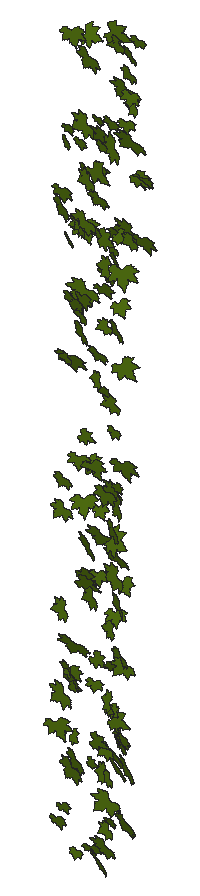
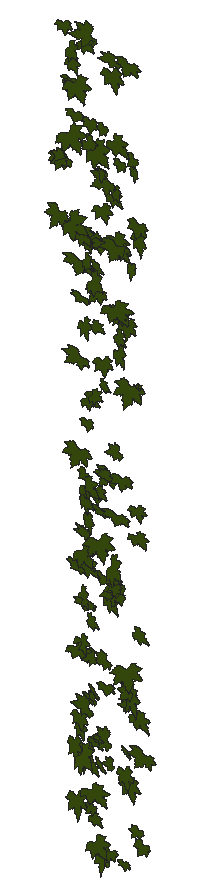
# SketchUp Ruby script. Lengths in inches.
U = 1.inch
M = Sketchup.active_model
def pt(a) = Geom::Point3d.new(a.map { |v| v * U })
def face(e, loops, mat)
  f = e.add_face(loops[0].map { |a| pt(a) })
  loops[1..].each { |l| e.add_face(l.map { |a| pt(a) }).erase! }
  f.material = f.back_material = mat if mat
  f
end
# faces: each face lists its corners as indices into pts; further lists are holes
def faces(e, pts, list, mat = nil) = list.each { |f| face(e, (f[0].is_a?(Array) ? f : [f]).map { |l| l.map { |i| pts[i] } }, mat) }
# xy, xz, yz: faces in a plane at the given z, y or x. An outline is a flat list of corners, or four numbers for a rectangle; further outlines are holes
def ring(l) = l.size == 4 ? [[l[0], l[1]], [l[2], l[1]], [l[2], l[3]], [l[0], l[3]]] : l.each_slice(2).to_a
def flat(e, list, mat, &to3) = list.each { |f| face(e, (f[0].is_a?(Array) ? f : [f]).map { |l| ring(l).map { |u, v| to3.(u, v) } }, mat) }
def xy(e, z, list, mat = nil) = flat(e, list, mat) { |x, y| [x, y, z] }
def xz(e, y, list, mat = nil) = flat(e, list, mat) { |x, z| [x, y, z] }
def yz(e, x, list, mat = nil) = flat(e, list, mat) { |y, z| [x, y, z] }
def lines(e, pts, list) = list.each { |a, b| e.add_line(pt(pts[a]), pt(pts[b])) }
# prism: a flat outline (further loops are holes) pulled along v
def prism(e, loops, v, mat = nil)
  f = face(e, loops, mat); d = Geom::Vector3d.new(v.map { |x| x * U })
  f.pushpull(f.normal.samedirection?(d) ? d.length : -d.length)
end
def box(e, o, s, mat = nil) = prism(e, [[o, [o[0] + s[0], o[1], o[2]], [o[0] + s[0], o[1] + s[1], o[2]], [o[0], o[1] + s[1], o[2]]]], [0, 0, s[2]], mat)
def at(x, y, z, deg = 0) = Geom::Transformation.translation(pt([x, y, z])) * Geom::Transformation.rotation(ORIGIN, Z_AXIS, deg.degrees)
def axes(o, x, y, z) = Geom::Transformation.new([*x, 0, *y, 0, *z, 0, *pt(o).to_a, 1])
def part(name) = M.definitions.add(name)
# library, detail: a bought-in or finely detailed component or shape, given as its bounding box
def library(name, o, s) = part(name).tap { |d| box(d.entities, o, s) }
def detail(e, o, s) = box(e.add_group.entities, o, s)
def put(e, d, t, mat = nil) = e.add_instance(d, t).tap { |i| i.material = mat if mat }
def group(e, t, mat = nil) = e.add_group.tap { |g| g.transformation = t; g.material = mat if mat }.entities
root = M.entities
M.materials.add("[Vegetation Blur 03]").color = [83, 114, 18]
c1 = part("ivy")
xy(c1.entities,0,[[0.782,0,0.786,0,0.787,0.005,0.789,0.009,0.821,0.072,0.875,0.147,1.001,0.272,1.073,0.331,1.137,0.363,1.178,0.379,1.223,0.384,1.272,0.383,1.311,0.374,1.36,0.355,1.399,0.334,1.491,0.285,1.541,0.244,1.583,0.199,1.617,0.15,1.64,0.128,1.662,0.115,1.717,0.105,1.745,0.093,1.784,0.054,1.819,0.057,1.854,0.064,1.882,0.075,1.896,0.074,1.91,0.071,1.937,0.063,1.964,0.053,1.99,0.038,2.016,0.015,2.034,0.002,2.04,0,2.038,0.003,2.036,0.007,2.033,0.038,2.036,0.068,2.045,0.1,2.055,0.116,2.064,0.123,2.077,0.129,2.088,0.129,2.106,0.132,2.118,0.13,2.179,0.132,2.207,0.133,2.225,0.133,2.242,0.138,2.22,0.162,2.207,0.186,2.206,0.213,2.212,0.236,2.228,0.262,2.247,0.274,2.298,0.283,2.355,0.294,2.37,0.296,2.376,0.295,2.377,0.3,2.377,0.303,2.385,0.329,2.411,0.37,2.426,0.392,2.449,0.407,2.511,0.426,2.561,0.444,2.619,0.466,2.589,0.469,2.561,0.476,2.501,0.5,2.449,0.516,2.424,0.523,2.401,0.535,2.377,0.556,2.372,0.568,2.36,0.575,2.268,0.586,2.225,0.592,2.207,0.599,2.194,0.61,2.143,0.65,2.13,0.664,2.122,0.682,2.123,0.7,2.13,0.719,2.148,0.75,2.17,0.781,2.195,0.807,2.221,0.828,2.284,0.874,2.291,0.88,2.288,0.887,2.276,0.9,2.267,0.916,2.265,0.933,2.273,0.967,2.292,1.002,2.313,1.03,2.334,1.054,2.348,1.067,2.358,1.074,2.363,1.076,2.362,1.081,2.35,1.094,2.347,1.11,2.35,1.143,2.359,1.18,2.385,1.254,2.415,1.324,2.448,1.393,2.45,1.4,2.446,1.398,2.44,1.394,2.427,1.383,2.402,1.36,2.376,1.339,2.345,1.324,2.305,1.309,2.282,1.303,2.273,1.306,2.245,1.294,2.212,1.287,2.187,1.291,2.163,1.301,2.142,1.316,2.134,1.327,2.124,1.325,2.09,1.292,2.053,1.259,2.014,1.234,1.973,1.215,1.954,1.21,1.931,1.208,1.909,1.212,1.893,1.22,1.879,1.233,1.872,1.248,1.867,1.281,1.864,1.319,1.821,1.258,1.773,1.197,1.726,1.141,1.698,1.121,1.679,1.116,1.666,1.117,1.647,1.122,1.632,1.129,1.62,1.141,1.617,1.154,1.617,1.219,1.621,1.254,1.623,1.268,1.623,1.281,1.618,1.314,1.606,1.346,1.603,1.375,1.607,1.403,1.603,1.467,1.599,1.499,1.605,1.525,1.614,1.552,1.629,1.577,1.635,1.589,1.629,1.587,1.618,1.582,1.596,1.566,1.581,1.556,1.568,1.552,1.557,1.55,1.545,1.553,1.531,1.562,1.522,1.572,1.504,1.591,1.486,1.611,1.474,1.631,1.457,1.666,1.455,1.684,1.457,1.698,1.452,1.715,1.444,1.728,1.424,1.754,1.419,1.772,1.423,1.786,1.434,1.819,1.444,1.848,1.446,1.855,1.44,1.861,1.43,1.867,1.386,1.904,1.349,1.948,1.326,1.973,1.31,1.995,1.288,2.048,1.284,2.153,1.287,2.254,1.284,2.255,1.282,2.253,1.278,2.247,1.274,2.237,1.266,2.216,1.226,2.125,1.208,2.076,1.184,2.033,1.155,1.984,1.135,1.942,1.111,1.899,1.083,1.861,1.053,1.85,1.059,1.83,1.061,1.809,1.056,1.79,1.049,1.767,1.04,1.749,1.018,1.733,0.994,1.726,0.942,1.734,0.95,1.6875,0.944,1.645,0.932,1.608,0.911,1.585,0.881,1.58,0.854,1.582,0.828,1.588,0.785,1.618,0.773,1.625,0.775,1.614,0.779,1.598,0.796,1.502,0.818,1.402,0.861,1.283,0.882,1.224,0.894,1.174,0.892,1.148,0.886,1.123,0.881,1.107,0.872,1.099,0.849,1.094,0.818,1.092,0.789,1.098,0.762,1.107,0.753,1.113,0.721,1.139,0.698,1.163,0.678,1.194,0.665,1.224,0.628,1.28,0.612,1.312,0.606,1.327,0.606,1.314,0.599,1.282,0.594,1.267,0.581,1.256,0.544,1.245,0.512,1.244,0.473,1.249,0.444,1.256,0.382,1.288,0.339,1.306,0.324,1.316,0.317,1.324,0.309,1.326,0.27,1.314,0.227,1.313,0.185,1.3125,0.152,1.317,0.122,1.328,0.092,1.345,0.073,1.353,0.079,1.338,0.092,1.308,0.117,1.249,0.13,1.215,0.139,1.164,0.147,1.148,0.157,1.136,0.163,1.122,0.174,1.086,0.177,1.067,0.182,1.054,0.186,1.043,0.191,1.038,0.211,1.028,0.237,1.005,0.25,0.974,0.253,0.96,0.25,0.944,0.242,0.914,0.243,0.906,0.249,0.902,0.26,0.894,0.289,0.88,0.307,0.873,0.322,0.862,0.364,0.799,0.403,0.738,0.431,0.709,0.439,0.691,0.441,0.678,0.4375,0.66,0.428,0.645,0.394,0.623,0.303,0.594,0.255,0.581,0.214,0.577,0.179,0.573,0.173,0.568,0.175,0.561,0.167,0.55,0.141,0.523,0.113,0.503,0.077,0.49,0.045,0.486,0.026,0.485,0.019,0.486,0.011,0.483,0,0.471,0.014,0.467,0.044,0.455,0.058,0.447,0.07,0.438,0.097,0.411,0.125,0.394,0.158,0.377,0.174,0.366,0.182,0.359,0.185,0.361,0.242,0.331,0.253,0.316,0.258,0.303,0.262,0.283,0.274,0.278,0.308,0.274,0.341,0.252,0.366,0.226,0.366,0.222,0.37,0.22,0.38,0.221,0.395,0.221,0.425,0.216,0.45,0.207,0.465,0.192,0.473,0.178,0.484,0.15,0.489,0.116,0.483,0.089,0.468,0.058,0.45,0.035,0.435,0.018,0.429,0.011,0.434,0.012,0.438,0.014,0.469,0.019,0.542,0.016,0.581,0.015,0.612,0.027,0.68,0.055,0.696,0.057,0.712,0.052,0.73,0.045,0.741,0.036,0.766,0.014]])
p = [[34.46,174.5,46.56],[34.375,174.5,46.56]]
lines(root,p,[[0,1]])
put(root,c1,axes([27.85,173.7,7.37],[0.37849,-0.06704,0.09137],[0.11442,0.06293,-0.30843],[-0.02244,-0.80977,-0.03153]),"[Vegetation Blur 03]")
put(root,c1,axes([27.48,173.7,12.03],[0.53376,0.03726,0.21952],[0.269,0.00727,-0.43585],[0.01776,-1.22992,0.00407]),"[Vegetation Blur 03]")
put(root,c1,axes([28.43,173.7,14.45],[0.42826,-0.11256,-0.35023],[-0.42906,0.04831,-0.35189],[-0.05529,-1.24664,0.01798]),"[Vegetation Blur 03]")
put(root,c1,axes([28.76,173.7,18.72],[0.19822,-0.13225,-0.36337],[-0.44645,0.06503,-0.16594],[-0.0552,-1.0008,0.03723]),"[Vegetation Blur 03]")
put(root,c1,axes([28.37,173.7,23.69],[0.40363,-0.02669,-0.22372],[-0.27442,-0.04788,-0.32887],[0.00236,-1.00289,0.02165]),"[Vegetation Blur 03]")
put(root,c1,axes([28.3,173.7,25.06],[0.38167,-0.01698,-0.15187],[-0.18516,0.0606,-0.31101],[-0.02031,-0.87168,-0.01866]),"[Vegetation Blur 03]")
put(root,c1,axes([28.29,173.7,39.18],[0.47471,-0.2198,-0.23723],[-0.27334,0.21714,-0.39597],[-0.14555,-1.12467,-0.03009]),"[Vegetation Blur 03]")
put(root,c1,axes([28.78,173.7,31.25],[0.13027,0.06294,-0.24641],[-0.30303,0.06322,-0.10416],[-0.01626,-0.67369,-0.0328]),"[Vegetation Blur 03]")
put(root,c1,axes([28.02,173.7,39.6],[0.49002,-0.06773,0.03255],[0.04203,0.06603,-0.39982],[-0.03013,-1.00954,-0.02833]),"[Vegetation Blur 03]")
put(root,c1,axes([28.22,173.7,8.02],[0.2717,-0.01326,0.11926],[0.14597,0.06528,-0.22036],[0.00938,-0.63148,-0.02528]),"[Vegetation Blur 03]")
put(root,c1,axes([28.79,173.7,15.5625],[0.44681,-0.13861,-0.40686],[-0.47518,0.33403,-0.36549],[-0.1651,-1.33648,-0.04915]),"[Vegetation Blur 03]")
put(root,c1,axes([28.47,173.7,16.84],[0.5883,0.12569,-0.22776],[-0.28567,0.25569,-0.4693],[0.00068,-1.31528,-0.113]),"[Vegetation Blur 03]")
put(root,c1,axes([28.69,173.7,42.33],[0.2858,-0.16556,-0.09391],[-0.1058,0.0991,-0.24194],[-0.0923,-0.62621,-0.01346]),"[Vegetation Blur 03]")
put(root,c1,axes([28.125,173.7,31.23],[0.67545,-0.01499,0.0047],[0.00705,0.26519,-0.54115],[-0.00605,-1.36446,-0.10523]),"[Vegetation Blur 03]")
put(root,c1,axes([28.76,173.7,37.39],[0.30779,-0.16022,-0.12096],[-0.12595,0.19898,-0.2549],[-0.11031,-0.67423,-0.04648]),"[Vegetation Blur 03]")
put(root,c1,axes([28.56,173.7,42.75],[0.27595,-0.07999,0.10883],[0.13684,0.05207,-0.2251],[-0.02378,-0.62852,-0.0325]),"[Vegetation Blur 03]")
put(root,c1,axes([28.71,173.7,10.78],[0.5571,-0.15804,-0.2532],[-0.30286,0.14883,-0.45846],[-0.10211,-1.30372,-0.02164]),"[Vegetation Blur 03]")
put(root,c1,axes([28.58,173.7,14.93],[0.31712,0.01449,0.22059],[0.2693,0.0595,-0.25849],[0.0241,-0.85537,-0.01424]),"[Vegetation Blur 03]")
put(root,c1,axes([28.42,173.7,47.6875],[0.52799,0.03971,0.1403],[0.17249,-0.03446,-0.43082],[0.01316,-1.14211,0.01788]),"[Vegetation Blur 03]")
put(root,c1,axes([28.71,173.7,34.47],[0.55471,-0.15442,-0.09413],[-0.10485,0.16405,-0.45388],[-0.08911,-1.1543,-0.05191]),"[Vegetation Blur 03]")
put(root,c1,axes([29.03,173.7,11.23],[0.48731,-0.17978,-0.24983],[-0.29064,0.21865,-0.40235],[-0.12987,-1.16387,-0.037]),"[Vegetation Blur 03]")
put(root,c1,axes([29.43,173.7,38.43],[0.27575,-0.07071,-0.32237],[-0.38727,0.16418,-0.22631],[-0.08498,-0.9776,-0.01469]),"[Vegetation Blur 03]")
put(root,c1,axes([28.98,173.7,14.13],[0.08923,-0.0651,0.22881],[0.28147,0.0622,-0.07033],[0.01942,-0.60224,-0.032]),"[Vegetation Blur 03]")
put(root,c1,axes([29.01,173.7,11.58],[0.08406,0.07505,0.23958],[0.28752,-0.16835,-0.0589],[-0.06954,-0.60538,0.04608]),"[Vegetation Blur 03]")
put(root,c1,axes([30.01,173.7,22.12],[0.10735,0.13666,-0.49936],[-0.59338,0.3622,-0.06937],[-0.16335,-1.22594,-0.07616]),"[Vegetation Blur 03]")
put(root,c1,axes([29.12,173.7,6.17],[0.29298,-0.03076,-0.00517],[-0.00747,-0.046,-0.2387],[-0.01442,-0.60127,0.01853]),"[Vegetation Blur 03]")
put(root,c1,axes([29.57,173.7,33.08],[0.29122,-0.09132,-0.34949],[-0.40801,0.28097,-0.238],[-0.13739,-1.02797,-0.034]),"[Vegetation Blur 03]")
put(root,c1,axes([29.72,173.7,33.86],[0.15958,-0.02123,-0.31626],[-0.37905,0.17205,-0.12921],[-0.08118,-0.84504,-0.01836]),"[Vegetation Blur 03]")
put(root,c1,axes([28.94,173.7,26.21],[0.45127,0.0715,0.00789],[0.01018,-0.0128,-0.36935],[0.0346,-0.92876,0.0057]),"[Vegetation Blur 03]")
put(root,c1,axes([29.4375,173.7,35.38],[0.53259,0.07407,-0.33493],[-0.4092,-0.06459,-0.43565],[0.04766,-1.38209,0.00241]),"[Vegetation Blur 03]")
put(root,c1,axes([29.81,173.7,43.9375],[0.36403,-0.06267,-0.40957],[-0.5016,0.04126,-0.29795],[-0.03412,-1.27511,0.01049]),"[Vegetation Blur 03]")
put(root,c1,axes([29.79,173.7,41.21],[0.19632,-0.0358,-0.23719],[-0.2774,0.19596,-0.15758],[-0.08838,-0.69459,-0.03223]),"[Vegetation Blur 03]")
put(root,c1,axes([29.29,173.7,42.38],[0.31483,-0.06922,0.03461],[0.04453,0.03834,-0.25772],[-0.03078,-0.65259,-0.01881]),"[Vegetation Blur 03]")
put(root,c1,axes([29.5625,173.7,38.875],[0.46325,-0.03451,-0.29794],[-0.36488,0.02419,-0.37832],[-0.02045,-1.21347,0.00093]),"[Vegetation Blur 03]")
put(root,c1,axes([30.04,173.7,41.03],[0.26205,-0.06963,-0.34462],[-0.42004,0.08964,-0.2156],[-0.05487,-1.01871,0.00458]),"[Vegetation Blur 03]")
put(root,c1,axes([29.57,173.7,20.43],[0.29824,-0.02143,-0.02343],[-0.02665,0.10046,-0.24043],[-0.01491,-0.60833,-0.03888]),"[Vegetation Blur 03]")
put(root,c1,axes([28.93,173.7,38.03],[0.60611,0.08882,0.16972],[0.20851,-0.00255,-0.49577],[0.04043,-1.31863,0.01239]),"[Vegetation Blur 03]")
put(root,c1,axes([29.09,173.7,24.07],[0.5345,0.11261,0.12686],[0.16236,-0.17388,-0.43135],[0.02823,-1.13219,0.07887]),"[Vegetation Blur 03]")
put(root,c1,axes([29.27,173.7,34.49],[0.44672,-0.11391,0.09884],[0.12385,0.0351,-0.3665],[-0.0489,-0.9518,-0.02535]),"[Vegetation Blur 03]")
put(root,c1,axes([29.48,173.7,26.99],[0.12471,-0.00455,0.29508],[0.36083,0.05141,-0.10146],[0.0229,-0.78534,-0.00835]),"[Vegetation Blur 03]")
put(root,c1,axes([29.64,173.7,47.26],[0.56003,-0.11483,-0.22477],[-0.26984,0.13286,-0.4585],[-0.07841,-1.27735,-0.02748]),"[Vegetation Blur 03]")
put(root,c1,axes([29.28,173.7,20.17],[0.35675,-0.1356,0.28151],[0.35114,0.1247,-0.28695],[-0.00453,-1.0135,-0.07297]),"[Vegetation Blur 03]")
put(root,c1,axes([30.2,173.7,19.94],[0.31943,-0.14813,-0.35105],[-0.42397,0.15166,-0.26703],[-0.10221,-1.09204,0.01053]),"[Vegetation Blur 03]")
put(root,c1,axes([29.53,173.7,47.25],[0.0857,0.17777,0.39101],[0.48593,0.02942,-0.07304],[0.02949,-1.0011,0.06729]),"[Vegetation Blur 03]")
put(root,c1,axes([29.3,173.7,19.58],[0.27593,-0.17427,0.39331],[0.48854,0.16147,-0.21704],[0.02723,-1.13128,-0.09157]),"[Vegetation Blur 03]")
put(root,c1,axes([29.71,173.7,6.52],[0.36983,0.02306,0.04655],[0.05424,0.13467,-0.29755],[0.02088,-0.75816,-0.05144]),"[Vegetation Blur 03]")
put(root,c1,axes([29.91,173.7,25.63],[0.07333,0.12212,0.31359],[0.38829,0.01811,-0.06159],[0.01986,-0.80476,0.0462]),"[Vegetation Blur 03]")
put(root,c1,axes([30.02,173.7,10.65],[0.09053,-0.05831,0.23092],[0.28382,-0.01925,-0.07488],[-0.01758,-0.61103,-0.01968]),"[Vegetation Blur 03]")
put(root,c1,axes([29.99,173.7,15.08],[0.35798,0.03491,0.00358],[0.00487,-0.0205,-0.29237],[0.01684,-0.73641,0.00831]),"[Vegetation Blur 03]")
put(root,c1,axes([30.1875,173.7,32.12],[0.41941,-0.00434,-0.1684],[-0.2031,0.16133,-0.33757],[-0.03648,-0.94822,-0.05667]),"[Vegetation Blur 03]")
put(root,c1,axes([29.59,173.7,25.9],[0.48195,0.00963,0.21143],[0.25864,0.04977,-0.39304],[0.01557,-1.12486,-0.01558]),"[Vegetation Blur 03]")
put(root,c1,axes([30.28,173.7,40.09],[0.40291,0.01111,-0.21009],[-0.25613,0.11786,-0.3262],[-0.02632,-0.9768,-0.04175]),"[Vegetation Blur 03]")
put(root,c1,axes([30.8,173.7,30.88],[0.08976,-0.09939,-0.28739],[-0.34963,0.10974,-0.07871],[-0.06393,-0.7397,0.02694]),"[Vegetation Blur 03]")
put(root,c1,axes([30.8,173.7,43.4],[0.2991,0.11532,-0.48246],[-0.59082,0.19391,-0.23668],[-0.05934,-1.34945,-0.07524]),"[Vegetation Blur 03]")
put(root,c1,axes([30.18,173.7,22.99],[0.56725,0.10726,-0.27566],[-0.34171,0.20149,-0.45603],[-0.00596,-1.34353,-0.0904]),"[Vegetation Blur 03]")
put(root,c1,axes([30.6875,173.7,7.27],[0.36107,0.086,-0.36328],[-0.44668,0.11955,-0.29126],[-0.01905,-1.17336,-0.0563]),"[Vegetation Blur 03]")
put(root,c1,axes([30.21,173.7,6.52],[0.54071,-0.2448,-0.19934],[-0.20803,0.34691,-0.44288],[-0.17473,-1.17061,-0.08956]),"[Vegetation Blur 03]")
put(root,c1,axes([30.29,173.7,38.13],[0.37713,0.02521,-0.05482],[-0.06814,0.09104,-0.30568],[0.00422,-0.78299,-0.03731]),"[Vegetation Blur 03]")
put(root,c1,axes([31.17,173.7,36.39],[0.11247,0.10768,-0.41349],[-0.50254,0.19726,-0.08297],[-0.08291,-1.04957,-0.05801]),"[Vegetation Blur 03]")
put(root,c1,axes([30.12,173.7,20.58],[0.38704,0.02073,0.09682],[0.11906,-0.06304,-0.31489],[0.00062,-0.83064,0.02631]),"[Vegetation Blur 03]")
put(root,c1,axes([30.3125,173.7,43.86],[0.29162,-0.09248,0.04712],[0.06325,0.07335,-0.23812],[-0.03677,-0.60733,-0.03593]),"[Vegetation Blur 03]")
put(root,c1,axes([30.08,173.7,15.95],[0.20869,-0.00294,0.30527],[0.37402,-0.00987,-0.17032],[-0.00489,-0.88135,0.00089]),"[Vegetation Blur 03]")
put(root,c1,axes([29.8,173.7,40.79],[0.38841,-0.03974,0.39058],[0.47889,0.01108,-0.31703],[-0.00798,-1.26829,-0.01501]),"[Vegetation Blur 03]")
put(root,c1,axes([30.6,173.7,41.65],[0.29613,-0.07388,-0.10232],[-0.12287,0.05638,-0.24327],[-0.04369,-0.65932,-0.00934]),"[Vegetation Blur 03]")
put(root,c1,axes([31.08,173.7,11.11],[0.14128,-0.20319,-0.29587],[-0.36071,0.14973,-0.1309],[-0.10517,-0.78653,0.05152]),"[Vegetation Blur 03]")
put(root,c1,axes([31.13,173.7,30.21],[0.08326,0.10722,-0.24971],[-0.31037,0.02564,-0.0672],[0.00148,-0.65202,-0.0437]),"[Vegetation Blur 03]")
put(root,c1,axes([30.19,173.7,11.61],[0.11289,-0.08937,0.40816],[0.50197,0.01041,-0.09212],[-0.00461,-1.05497,-0.03549]),"[Vegetation Blur 03]")
put(root,c1,axes([30.62,173.7,42.74],[0.29319,-0.08212,-0.05398],[-0.06371,0.04494,-0.24127],[-0.04367,-0.61685,-0.01039]),"[Vegetation Blur 03]")
put(root,c1,axes([30.32,173.7,23.81],[0.27283,0.0757,0.1916],[0.23721,-0.13013,-0.2169],[-0.01401,-0.72914,0.0586]),"[Vegetation Blur 03]")
put(root,c1,axes([31.1,173.7,33.78],[0.19574,-0.01438,-0.25163],[-0.30815,-0.03945,-0.1593],[0.01245,-0.75048,0.0132]),"[Vegetation Blur 03]")
put(root,c1,axes([30.87,173.7,9.83],[0.47968,0.02946,-0.35016],[-0.4281,-0.06549,-0.39149],[0.03188,-1.32271,0.01158]),"[Vegetation Blur 03]")
put(root,c1,axes([31.37,173.7,36.9],[0.09556,-0.13792,-0.34176],[-0.41905,0.10501,-0.08471],[-0.06516,-0.87761,0.04357]),"[Vegetation Blur 03]")
put(root,c1,axes([30.97,173.7,12.26],[0.31122,-0.06083,-0.21678],[-0.26689,-0.02709,-0.25402],[-0.01391,-0.84152,0.02385]),"[Vegetation Blur 03]")
put(root,c1,axes([31.12,173.7,8.21],[0.24157,-0.07416,-0.2538],[-0.31175,0.01688,-0.19842],[-0.02861,-0.81014,0.0191]),"[Vegetation Blur 03]")
put(root,c1,axes([30.3125,173.7,35.19],[0.40086,-0.0573,0.17483],[0.21594,0.13183,-0.32299],[0.00594,-0.92596,-0.0568]),"[Vegetation Blur 03]")
put(root,c1,axes([30.53,173.7,25.18],[0.52679,-0.06661,-0.07919],[-0.09633,0.02908,-0.43069],[-0.03439,-1.10187,-0.00658]),"[Vegetation Blur 03]")
put(root,c1,axes([31.51,173.7,14.77],[0.05013,-0.17245,-0.31461],[-0.38087,0.18721,-0.05657],[-0.1028,-0.77773,0.05615]),"[Vegetation Blur 03]")
put(root,c1,axes([31.61,173.7,11.78],[0.15704,0.2136,-0.46973],[-0.57168,0.3147,-0.1048],[-0.12334,-1.18664,-0.11235]),"[Vegetation Blur 03]")
put(root,c1,axes([31.21,173.7,10.8],[0.21308,-0.10262,-0.22404],[-0.27243,0.07685,-0.17812],[-0.0602,-0.71097,0.01308]),"[Vegetation Blur 03]")
put(root,c1,axes([31.53,173.7,18.47],[0.09612,-0.08439,-0.33414],[-0.40558,0.12635,-0.08273],[-0.06933,-0.85613,0.02072]),"[Vegetation Blur 03]")
put(root,c1,axes([31.53,173.7,25.61],[0.20248,0.05039,-0.42079],[-0.51446,0.11243,-0.16277],[-0.042,-1.13431,-0.03483]),"[Vegetation Blur 03]")
put(root,c1,axes([30.62,173.7,37.32],[0.06821,0.02412,0.38984],[0.47536,-0.1037,-0.05439],[-0.04826,-0.98747,0.01524]),"[Vegetation Blur 03]")
put(root,c1,axes([31.54,173.7,29.97],[0.16222,0.03807,-0.33908],[-0.41557,-0.02093,-0.13279],[0.01621,-0.91758,-0.01104]),"[Vegetation Blur 03]")
put(root,c1,axes([31.58,173.7,37.18],[0.08292,0.05054,-0.29306],[-0.34577,0.22171,-0.05915],[-0.09993,-0.72524,-0.0385]),"[Vegetation Blur 03]")
put(root,c1,axes([31.41,173.7,22.22],[0.33518,0.12814,-0.38098],[-0.46864,0.20726,-0.26366],[-0.04654,-1.16428,-0.08887]),"[Vegetation Blur 03]")
put(root,c1,axes([31.49,173.7,43.36],[0.33503,-0.17484,-0.44401],[-0.53885,0.1655,-0.28108],[-0.11328,-1.30432,0.02385]),"[Vegetation Blur 03]")
put(root,c1,axes([31.91,173.7,25.03],[0.10156,-0.07064,-0.4993],[-0.59327,0.30784,-0.08723],[-0.15326,-1.23847,0.0068]),"[Vegetation Blur 03]")
put(root,c1,axes([31,173.7,44.1],[0.37183,-0.05449,-0.06268],[-0.07386,0.08152,-0.30299],[-0.03383,-0.77703,-0.02739]),"[Vegetation Blur 03]")
put(root,c1,axes([31.64,173.7,21.5],[0.29364,-0.08887,-0.43973],[-0.53794,0.07502,-0.24166],[-0.05272,-1.26047,0.01662]),"[Vegetation Blur 03]")
put(root,c1,axes([31.02,173.7,13.67],[0.05383,0.00628,0.24765],[0.29967,-0.10102,-0.04299],[-0.04781,-0.62607,0.00942]),"[Vegetation Blur 03]")
put(root,c1,axes([31.5,173.7,38.52],[0.25146,0.10077,-0.27244],[-0.33679,0.12568,-0.19974],[-0.01997,-0.85077,-0.06178]),"[Vegetation Blur 03]")
put(root,c1,axes([30.93,173.7,15.97],[0.19108,-0.09038,0.20852],[0.25839,0.11931,-0.14958],[0.021,-0.6456,-0.05683]),"[Vegetation Blur 03]")
put(root,c1,axes([31.4,173.7,37.79],[0.23501,-0.07019,-0.1629],[-0.19555,0.08472,-0.19365],[-0.05258,-0.62881,-0.00791]),"[Vegetation Blur 03]")
put(root,c1,axes([31.33,173.7,23.66],[0.37161,-0.21861,-0.25288],[-0.28876,0.23657,-0.31481],[-0.15463,-0.96714,-0.01984]),"[Vegetation Blur 03]")
put(root,c1,axes([30.96,173.7,8.28],[0.2775,-0.12673,0.11481],[0.14869,0.07236,-0.22682],[-0.03837,-0.63611,-0.04867]),"[Vegetation Blur 03]")
put(root,c1,axes([31.67,173.7,48.4],[0.21316,0.03069,-0.31446],[-0.38542,0.04396,-0.17335],[-0.01149,-0.90506,-0.01908]),"[Vegetation Blur 03]")
put(root,c1,axes([31.77,173.7,19.84],[0.20676,-0.07941,-0.38547],[-0.44776,0.31453,-0.17016],[-0.15519,-1.01328,-0.02261]),"[Vegetation Blur 03]")
put(root,c1,axes([31.5,173.7,33.8],[0.3273,-0.0909,-0.29956],[-0.34726,0.27044,-0.26563],[-0.12681,-0.97518,-0.04574]),"[Vegetation Blur 03]")
put(root,c1,axes([31.18,173.7,11.71],[0.5589,-0.19272,-0.25961],[-0.28238,0.39595,-0.45114],[-0.17385,-1.26271,-0.10184]),"[Vegetation Blur 03]")
put(root,c1,axes([31.27,173.7,28.42],[0.33014,-0.06379,-0.05513],[-0.06679,0.02302,-0.2706],[-0.03261,-0.69306,-0.00391]),"[Vegetation Blur 03]")
put(root,c1,axes([31.16,173.7,13.71],[0.13106,0.04715,0.22271],[0.27208,-0.09295,-0.10355],[-0.03102,-0.61597,0.03267]),"[Vegetation Blur 03]")
put(root,c1,axes([31.0625,173.7,18.91],[0.41222,0.08825,0.09854],[0.12607,-0.1297,-0.333],[0.02291,-0.87434,0.05934]),"[Vegetation Blur 03]")
put(root,c1,axes([30.97,173.7,21.91],[0.09143,0.21564,0.47102],[0.58317,-0.16267,-0.06368],[-0.06308,-1.19139,0.09395]),"[Vegetation Blur 03]")
put(root,c1,axes([31.66,173.7,17.27],[0.3587,-0.08547,-0.26789],[-0.31864,0.17898,-0.29317],[-0.08908,-0.98439,-0.03004]),"[Vegetation Blur 03]")
put(root,c1,axes([31.74,173.7,12.8],[0.31159,-0.10577,-0.25159],[-0.29051,0.23223,-0.255],[-0.11522,-0.87155,-0.03742]),"[Vegetation Blur 03]")
put(root,c1,axes([30.96,173.7,47.86],[0.15219,-0.0035,0.49259],[0.60198,0.09401,-0.12377],[0.04388,-1.27745,-0.01046]),"[Vegetation Blur 03]")
put(root,c1,axes([31.7,173.7,46.33],[0.49914,0.06889,-0.35402],[-0.43405,0.1716,-0.40237],[-0.0297,-1.34994,-0.06922]),"[Vegetation Blur 03]")
put(root,c1,axes([32.34,173.7,39.19],[0.20681,0.14961,-0.50522],[-0.62308,0.08477,-0.16594],[-0.01632,-1.34039,-0.06689]),"[Vegetation Blur 03]")
put(root,c1,axes([31.41,173.7,25.4],[0.23912,-0.07387,0.13682],[0.16931,0.00875,-0.19635],[-0.02693,-0.60087,-0.01968]),"[Vegetation Blur 03]")
put(root,c1,axes([31.18,173.7,12.95],[0.10403,0.04174,0.45584],[0.55849,-0.05312,-0.08413],[-0.02168,-1.16792,0.02012]),"[Vegetation Blur 03]")
put(root,c1,axes([31.73,173.7,16.82],[0.41939,0.05909,-0.24373],[-0.29711,-0.06483,-0.343],[0.04165,-1.05748,0.00741]),"[Vegetation Blur 03]")
put(root,c1,axes([31.4,173.7,37.9],[0.15956,0.10306,0.24419],[0.30313,-0.02658,-0.13017],[0.01203,-0.69728,0.04105]),"[Vegetation Blur 03]")
put(root,c1,axes([31.62,173.7,13.1875],[0.45644,-0.12973,-0.15733],[-0.18474,0.13729,-0.3748],[-0.08372,-1.01031,-0.03073]),"[Vegetation Blur 03]")
put(root,c1,axes([31.32,173.7,34.54],[0.32504,0.10399,0.20827],[0.26014,-0.12611,-0.26052],[0.00118,-0.84097,0.06482]),"[Vegetation Blur 03]")
put(root,c1,axes([32.0625,173.7,43.73],[0.44413,0.17265,-0.41061],[-0.51006,0.15289,-0.35736],[-0.00095,-1.3725,-0.09146]),"[Vegetation Blur 03]")
put(root,c1,axes([31.68,173.7,9.05],[0.5663,-0.16171,-0.26651],[-0.30497,0.30432,-0.46069],[-0.14072,-1.31032,-0.0741]),"[Vegetation Blur 03]")
put(root,c1,axes([31.12,173.7,36.52],[0.63449,0.08244,0.15008],[0.18708,-0.13099,-0.51549],[0.02055,-1.35306,0.05905]),"[Vegetation Blur 03]")
put(root,c1,axes([32.41,173.7,47.91],[0.1485,0.06744,-0.32773],[-0.39216,0.22625,-0.11103],[-0.09244,-0.8515,-0.05546]),"[Vegetation Blur 03]")
put(root,c1,axes([31.22,173.7,26.7],[0.61927,-0.03223,0.11526],[0.14207,0.12094,-0.50313],[-0.00213,-1.30144,-0.04961]),"[Vegetation Blur 03]")
put(root,c1,axes([31.96,173.7,11.85],[0.48214,-0.22782,-0.28181],[-0.31501,0.32234,-0.39997],[-0.17959,-1.177,-0.05499]),"[Vegetation Blur 03]")
put(root,c1,axes([31.27,173.7,31.27],[0.38223,0.09975,0.36551],[0.44923,0.00523,-0.31313],[0.03341,-1.2116,0.02874]),"[Vegetation Blur 03]")
put(root,c1,axes([31.78,173.7,44.17],[0.36239,0.03439,0.0325],[0.04011,-0.01114,-0.29602],[0.01602,-0.75014,0.00588]),"[Vegetation Blur 03]")
put(root,c1,axes([32.21,173.7,47.07],[0.31224,-0.04153,-0.22289],[-0.2695,0.10455,-0.25454],[-0.04857,-0.84719,-0.02048]),"[Vegetation Blur 03]")
put(root,c1,axes([31.61,173.7,20.41],[0.30062,0.06409,0.25513],[0.31279,-0.14376,-0.23982],[-0.02918,-0.88082,0.05771]),"[Vegetation Blur 03]")
put(root,c1,axes([32.47,173.7,38.62],[0.2286,-0.00259,-0.27195],[-0.33307,0.02295,-0.18652],[-0.00991,-0.83122,-0.0043]),"[Vegetation Blur 03]")
put(root,c1,axes([32.91,173.7,45.72],[0.11758,-0.14394,-0.33997],[-0.41694,0.10295,-0.1029],[-0.06765,-0.88473,0.04334]),"[Vegetation Blur 03]")
put(root,c1,axes([32.04,173.7,45.8],[0.42779,-0.01722,0.00276],[0.0027,-0.07154,-0.34805],[-0.00862,-0.87743,0.02832]),"[Vegetation Blur 03]")
put(root,c1,axes([32.5625,173.7,48.75],[0.32819,0.01887,-0.10221],[-0.12554,0.06541,-0.2666],[-0.0028,-0.71988,-0.0269]),"[Vegetation Blur 03]")
put(root,c1,axes([32.33,173.7,41.29],[0.29759,0.01634,0.29239],[0.3571,0.0663,-0.24267],[0.02985,-0.95609,-0.01183]),"[Vegetation Blur 03]")
put(root,c1,axes([32.63,173.7,41.7],[0.43208,-0.00485,-0.01137],[-0.01346,0.125,-0.34915],[-0.00429,-0.88078,-0.04949]),"[Vegetation Blur 03]")
put(root,c1,axes([32.53,173.7,38.58],[0.54527,-0.10858,0.11727],[0.14945,0.14116,-0.4423],[-0.03309,-1.15173,-0.06527]),"[Vegetation Blur 03]")
